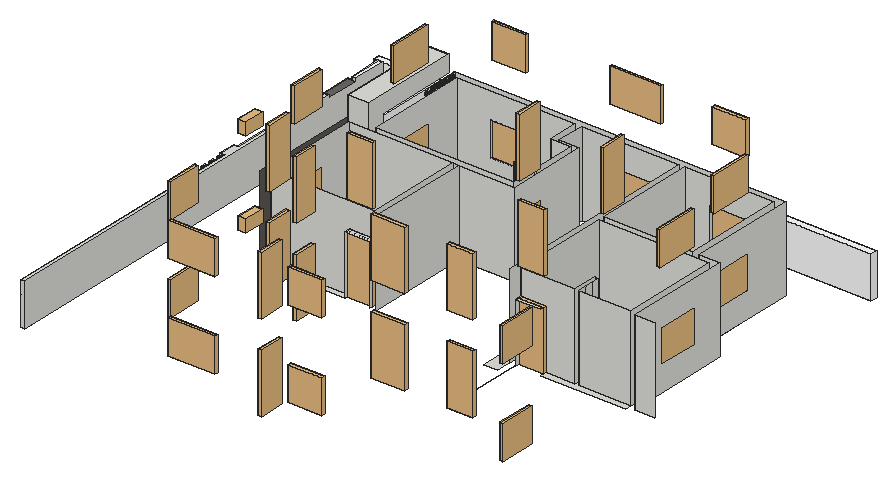
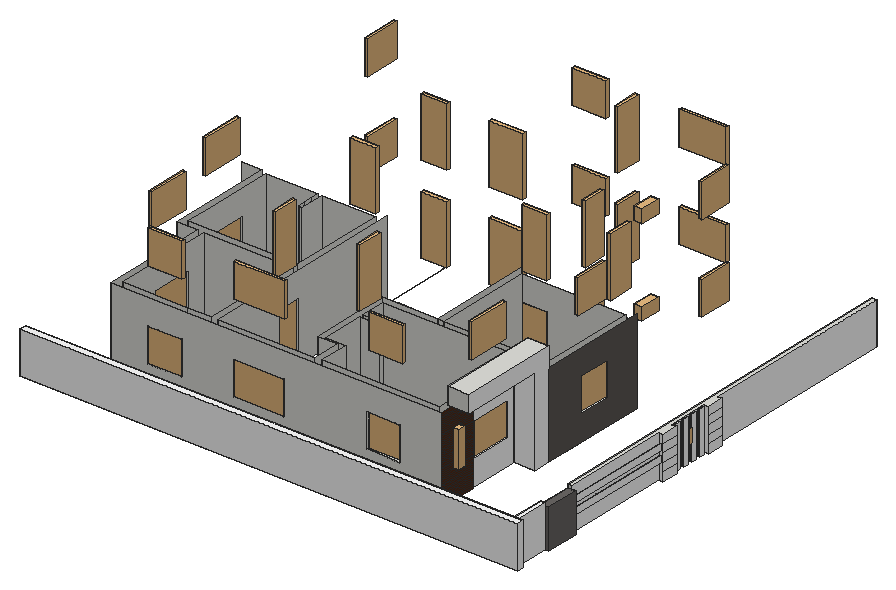
# SketchUp Ruby script. Lengths in inches.
U = 1.inch
M = Sketchup.active_model
def pt(a) = Geom::Point3d.new(a.map { |v| v * U })
def face(e, loops, mat)
  f = e.add_face(loops[0].map { |a| pt(a) })
  loops[1..].each { |l| e.add_face(l.map { |a| pt(a) }).erase! }
  f.material = f.back_material = mat if mat
  f
end
# faces: each face lists its corners as indices into pts; further lists are holes
def faces(e, pts, list, mat = nil) = list.each { |f| face(e, (f[0].is_a?(Array) ? f : [f]).map { |l| l.map { |i| pts[i] } }, mat) }
# xy, xz, yz: faces in a plane at the given z, y or x. An outline is a flat list of corners, or four numbers for a rectangle; further outlines are holes
def ring(l) = l.size == 4 ? [[l[0], l[1]], [l[2], l[1]], [l[2], l[3]], [l[0], l[3]]] : l.each_slice(2).to_a
def flat(e, list, mat, &to3) = list.each { |f| face(e, (f[0].is_a?(Array) ? f : [f]).map { |l| ring(l).map { |u, v| to3.(u, v) } }, mat) }
def xy(e, z, list, mat = nil) = flat(e, list, mat) { |x, y| [x, y, z] }
def xz(e, y, list, mat = nil) = flat(e, list, mat) { |x, z| [x, y, z] }
def yz(e, x, list, mat = nil) = flat(e, list, mat) { |y, z| [x, y, z] }
def lines(e, pts, list) = list.each { |a, b| e.add_line(pt(pts[a]), pt(pts[b])) }
# prism: a flat outline (further loops are holes) pulled along v
def prism(e, loops, v, mat = nil)
  f = face(e, loops, mat); d = Geom::Vector3d.new(v.map { |x| x * U })
  f.pushpull(f.normal.samedirection?(d) ? d.length : -d.length)
end
def box(e, o, s, mat = nil) = prism(e, [[o, [o[0] + s[0], o[1], o[2]], [o[0] + s[0], o[1] + s[1], o[2]], [o[0], o[1] + s[1], o[2]]]], [0, 0, s[2]], mat)
def at(x, y, z, deg = 0) = Geom::Transformation.translation(pt([x, y, z])) * Geom::Transformation.rotation(ORIGIN, Z_AXIS, deg.degrees)
def axes(o, x, y, z) = Geom::Transformation.new([*x, 0, *y, 0, *z, 0, *pt(o).to_a, 1])
def part(name) = M.definitions.add(name)
# library, detail: a bought-in or finely detailed component or shape, given as its bounding box
def library(name, o, s) = part(name).tap { |d| box(d.entities, o, s) }
def detail(e, o, s) = box(e.add_group.entities, o, s)
def put(e, d, t, mat = nil) = e.add_instance(d, t).tap { |i| i.material = mat if mat }
def group(e, t, mat = nil) = e.add_group.tap { |g| g.transformation = t; g.material = mat if mat }.entities
root = M.entities
M.materials.add("Bricks A03 100cm").color = [95, 90, 86]
M.materials.add("Cl-3460 22.24cm").color = [255, 255, 255]
M.materials.add("Manhattan Creative Coating MD 1125B 26.44cm").color = [255, 255, 255]
M.materials.add("Paint White Matte 002 0.02cm").color = [255, 255, 255]
M.materials.add("Pp-1846-msg 17.72cm").color = [255, 255, 255]
M.materials.add("Stone C 250cm").color = [107, 104, 102]
M.materials.add("Wintan - wpa36452 29.79cm").color = [255, 255, 255]
M.materials.add("Wintan - wpa36452 29.79cm\#1").color = [255, 255, 255]
M.materials.add("Wood 011 26.84cm").color = [255, 255, 255]
M.materials.add("Wood Mahogany 33-46 100cm").color = [84, 42, 21]
c1 = library("Window Crafter Sliding 3",[0,-0.55,0],[48,4.49,48])
c2 = library("usa interior dubla",[9.3,83.61,0],[74.77,5.52,82.68])
c3 = library("Window Crafter Awning 2",[0,-9.5,0],[29,11.27,18])
c4 = library("Door 243 065",[-19.36,-2.49,0],[38.72,4.98,81.96])
c5 = library("Door 243 074",[-20.11,-2.41,0],[40.22,4.82,86.63])
c6 = part("*U28\#1")
p = [[0,0,0],[0,36,0],[-1.75,36,0],[-1.75,0,0],[-2.26,35.93,0],[-4.51,35.72,0],
  [-6.75,35.36,0],[-8.95,34.87,0],[-11.125,34.24,0],[-13.25,33.47,0],[-15.33,32.57,0],[-17.34,31.55,0],
  [-19.29,30.4,0],[-21.16,29.125,0],[-22.95,27.74,0],[-24.64,26.24,0],[-26.24,24.64,0],[-27.74,22.95,0],
  [-29.125,21.16,0],[-30.4,19.29,0],[-31.55,17.34,0],[-32.57,15.33,0],[-33.47,13.25,0],[-34.24,11.125,0],
  [-34.87,8.95,0],[-35.36,6.75,0],[-35.72,4.51,0],[-35.93,2.26,0],[-36,0,0],[0,-6,0],
  [-36,-6,0]]
lines(c6.entities,p,[[0,1],[1,2],[2,3],[3,0],[1,4],[4,5],[5,6],[6,7],[7,8],[8,9],[9,10],[10,11],
  [11,12],[12,13],[13,14],[14,15],[15,16],[16,17],[17,18],[18,19],[19,20],[20,21],[21,22],[22,23],
  [23,24],[24,25],[25,26],[26,27],[27,28],[0,29],[28,30]])
c7 = part("Rectangular post")
xy(c7.entities,0,[[0,0,3.4375,7.625]])
xy(c7.entities,60,[[0,0,3.4375,7.625]],"Paint White Matte 002 0.02cm")
xz(c7.entities,0,[[0,0,3.4375,60]],"Paint White Matte 002 0.02cm")
xz(c7.entities,7.625,[[0,0,3.4375,60]],"Paint White Matte 002 0.02cm")
yz(c7.entities,0,[[0,0,7.625,60]],"Paint White Matte 002 0.02cm")
yz(c7.entities,3.4375,[[0,0,7.625,60]])
c8 = library("Group\#37",[0,0,0],[10.9375,10.44,50.62])
c9 = part("*U29\#1")
p = [[0,0,0],[0,-36,0],[-1.75,-36,0],[-1.75,0,0],[-36,0,0],[-35.93,-2.26,0],
  [-35.72,-4.51,0],[-35.36,-6.75,0],[-34.87,-8.95,0],[-34.24,-11.125,0],[-33.47,-13.25,0],[-32.57,-15.33,0],
  [-31.55,-17.34,0],[-30.4,-19.29,0],[-29.125,-21.16,0],[-27.74,-22.95,0],[-26.24,-24.64,0],[-24.64,-26.24,0],
  [-22.95,-27.74,0],[-21.16,-29.125,0],[-19.29,-30.4,0],[-17.34,-31.55,0],[-15.33,-32.57,0],[-13.25,-33.47,0],
  [-11.125,-34.24,0],[-8.95,-34.87,0],[-6.75,-35.36,0],[-4.51,-35.72,0],[-2.26,-35.93,0],[0,6,0],
  [-36,6,0]]
lines(c9.entities,p,[[0,1],[1,2],[2,3],[3,0],[4,5],[5,6],[6,7],[7,8],[8,9],[9,10],[10,11],[11,12],
  [12,13],[13,14],[14,15],[15,16],[16,17],[17,18],[18,19],[19,20],[20,21],[21,22],[22,23],[23,24],
  [24,25],[25,26],[26,27],[27,28],[28,1],[0,29],[4,30]])
c10 = part("Group\#34")
box(c10.entities,[0,0,0],[3,153.5625,9])
c11 = library("Dining Set - 36 x 72 in.\#3",[-45.5,-27.5,0],[91,55,0.01])
c12 = library("Range-Oven - 30 in top\#2",[0,-26,0],[30,26,0.01])
xy(root,0,[[511.31,291.22,511.37,550.5],[482.12,382.5,502.31,449.24],[547.31,403.5,547.31,412.5,587.97,412.5,587.97,447.375,592.97,447.375,592.97,412.5,667.31,412.5,667.31,403.5],[148.31,403.63,148.31,454.3,157.31,454.3,157.31,412.5,268.31,412.5,268.31,403.63],[268.31,403.63,268.43,412.5],
  [645.22,465.17,654.6,479.125,654.6,473.03,665.48,473.03,665.48,492.22,655.11,492.22,655.11,496.88,665.48,496.88,665.48,516.07,655.11,516.07,655.11,523.17,667.17,523.17,667.17,465.17],[654.6,479.125,654.6,479.87,655.11,479.87],[640.18,479.87,640.02,480.43,639.96,480.67,640.32,480.3,640.74,479.87],[654.6,479.87,655.11,492.22],[639.96,480.67,639.9,480.74,639.8,480.84,639.73,481,639.51,481.57,639.29,482.13,638.83,483.27,638.6,483.83,638.37,484.4,638.13,484.96,637.89,485.51,637.64,486.07,637.39,486.62,637.14,487.16,636.88,487.7,636.34,488.76,636.0625,489.27,635.78,489.78,635.48,490.29,635.18,490.78,634.875,491.26,634.56,491.73,634.23,492.2,633.89,492.65,633.55,493.08,633.19,493.51,632.83,493.92,632.45,494.32,632.0625,494.7,631.66,495.07,631.25,495.42,630.83,495.75,630.39,496.07,629.9375,496.37,629.47,496.65,628.99,496.92,628.5,497.16,627.99,497.38,627.47,497.59,626.93,497.77,626.38,497.94,625.82,498.09,625.25,498.23,624.68,498.36,623.52,498.6,622.36,498.82,620.65,499.15,619.55,499.41,619.02,499.55,618.51,499.7,618.01,499.87,617.53,500.06,617.07,500.26,616.63,500.49,616.22,500.73,615.83,501.01,615.46,501.3,615.11,501.61,614.79,501.95,614.49,502.31,614.21,502.68,613.94,503.08,613.7,503.49,613.48,503.92,613.27,504.37,613.08,504.84,612.91,505.32,612.76,505.82,612.62,506.33,612.5,506.86,612.39,507.4,612.3,507.95,612.22,508.52,612.15,509.1,612.09,509.7,612.05,510.3,612.02,510.91,611.99,511.54,611.98,512.17,611.98,512.82,611.99,513.47,612,514.13,612.02,514.8,612.05,515.47,612.09,516.15,612.17,517.53,612.23,518.22,612.28,518.92,612.4,520.33,612.47,521.04,612.53,521.75,612.67,523.17,616.25,523.17,616.22,522.54,616.14,521.28,616.1,520.66,616.07,520.03,616.01,518.79,615.99,518.18,615.97,517.5625,615.95,516.95,615.94,516.35,615.94,515.15,615.95,514.5625,615.97,513.98,615.99,513.4,616.03,512.83,616.07,512.27,616.125,511.71,616.1875,511.17,616.26,510.63,616.34,510.1,616.4375,509.58,616.55,509.07,616.67,508.57,616.8,508.08,616.95,507.6,617.11,507.14,617.29,506.68,617.49,506.24,617.69,505.81,617.92,505.4,618.16,505,618.42,504.61,618.7,504.24,619,503.88,619.32,503.54,619.65,503.21,620.01,502.9,620.39,502.61,620.78,502.33,621.2,502.07,621.63,501.82,622.08,501.59,622.55,501.36,623.02,501.14,623.51,500.94,624,500.73,624.5,500.53,625,500.34,625.51,500.14,626.02,499.95,627.04,499.55,627.55,499.34,628.05,499.13,628.54,498.91,629.03,498.6875,629.5,498.45,629.96,498.2,630.41,497.93,630.85,497.65,631.27,497.36,631.67,497.05,632.07,496.73,632.45,496.4,632.8125,496.05,633.17,495.69,633.51,495.32,633.84,494.9375,634.16,494.54,634.47,494.14,634.76,493.72,635.05,493.29,635.33,492.86,635.6,492.41,635.86,491.96,636.11,491.5,636.35,491.02,636.81,490.06,637.03,489.5625,637.24,489.0625,637.45,488.55,637.65,488.04,638.03,487,638.39,485.94,638.57,485.4,638.74,484.86,638.91,484.31,639.07,483.76,639.24,483.21,639.4,482.66,639.56,482.1,639.71,481.55,639.87,480.99],
  [654.6,496.88,655.11,516.07],[148.31,502.3,148.31,559.5,178.31,559.5,178.31,594.58,187.31,594.58,187.31,559.5,392.57,559.5,392.57,550.5,157.31,550.5,157.31,502.3],[392.57,550.5,502.31,559.5],[214.32,559.5,281.06,580.44],[637.31,586.67,646.31,646.67],
  [502.31,595.5,502.31,703.5,473.12,703.5,473.12,712.5,546.3125,712.5,546.3125,703.5,511.31,703.5,511.31,595.5],[355.31,595.72,355.31,600.44,383.57,600.44,383.57,660.44,355.31,660.44,355.31,703.5,284.58,703.5,284.58,712.5,401.12,712.5,401.12,703.5,364.31,703.5,364.31,664.25,392.57,664.25,392.57,595.72],[637.31,646.67,637.31,703.5,594.3125,703.5,594.3125,712.5,646.31,712.5,646.31,646.67],[178.31,654.58,178.31,712.5,236.58,712.5,236.58,703.5,187.31,703.5,187.31,654.58],[401.12,703.5,473.12,712.5],
  [718.31,763.5,727.31,772.5],[373.31,769.5,400.94,772.5],[400.94,769.5,403.94,772.5],[447.58,769.5,450.58,772.5],[450.58,769.5,490.31,772.5]])
xy(root,36,[[667.31,453.9,676.31,513.9],[148.31,454.3,157.31,502.3],[637.31,586.67,646.31,646.67],[178.31,594.58,187.31,654.58],[236.58,703.5,284.58,712.5],
  [401.12,703.5,473.12,712.5],[546.3125,703.5,594.3125,712.5]])
xy(root,84,[[511.31,403.5,547.31,412.5],[268.31,403.63,304.31,412.5],[667.31,453.9,676.31,513.9],[148.31,454.3,157.31,502.3],[383.57,559.5,392.57,595.72],
  [502.31,559.5,511.31,595.5],[637.31,586.67,646.31,646.67],[178.31,594.58,187.31,654.58],[236.58,703.5,284.58,712.5],[401.12,703.5,473.12,712.5],
  [546.3125,703.5,594.3125,712.5]])
xz(root,408.16,[[676.31,0,704.78,120]])
xz(root,412.5,[[157.31,0,157.31,120,304.31,120,304.31,84,268.31,84,268.31,0],[547.31,0,547.31,84,511.31,84,511.31,120,587.97,120,587.97,0],[592.97,0,667.31,120]])
xz(root,447.375,[[587.97,0,592.97,120]])
xz(root,453.9,[[667.31,36,676.31,84]])
xz(root,454.3,[[148.31,36,157.31,84]])
xz(root,502.3,[[148.31,36,157.31,84]])
xz(root,513.9,[[667.31,36,676.31,84]])
xz(root,550.5,[[157.31,0,304.31,120],[304.31,0,313.31,120],[313.31,0,392.57,120],[511.31,0,511.37,120],[511.37,0,667.31,120]])
xz(root,559.5,[[187.31,0,187.31,120,383.57,120,383.57,84,392.57,84,392.57,0],[502.31,0,502.31,84,511.31,84,511.31,120,637.31,120,637.31,0],[646.31,0,676.31,120]])
xz(root,559.5,[[148.31,0,178.31,120]],"Pp-1846-msg 17.72cm")
xz(root,586.67,[[637.31,36,646.31,84]])
xz(root,594.58,[[178.31,36,187.31,84]])
xz(root,595.5,[[502.31,0,511.31,84]])
xz(root,595.72,[[355.31,0,392.57,0,392.57,84,383.57,84,383.57,120,355.31,120]])
xz(root,600.44,[[355.31,0,383.57,120]])
xz(root,646.67,[[637.31,36,646.31,84]])
xz(root,654.58,[[178.31,36,187.31,84]])
xz(root,660.44,[[355.31,0,383.57,120]])
xz(root,664.25,[[364.31,0,392.57,120]])
xz(root,703.5,[[[187.31,0,355.31,120],[236.58,36,284.58,84]],[[364.31,0,502.31,120],[401.12,36,473.12,84]],[511.31,0,546.3125,120],[546.3125,0,594.3125,36],[594.3125,0,637.31,0,637.31,120,546.3125,120,546.3125,84,594.3125,84]])
xz(root,712.5,[[[178.31,0,646.31,120],[401.12,36,473.12,84],[236.58,36,284.58,84],[546.3125,36,594.3125,84]]])
yz(root,148.31,[[[403.63,0,559.5,120],[454.3,36,502.3,84]]],"Bricks A03 100cm")
yz(root,157.31,[[412.5,0,454.3,0,454.3,84,502.3,84,502.3,36,454.3,36,454.3,0,550.5,0,550.5,120,412.5,120]])
yz(root,178.31,[[[559.5,0,712.5,120],[594.58,36,654.58,84]]],"Pp-1846-msg 17.72cm")
yz(root,187.31,[[[559.5,0,703.5,120],[594.58,36,654.58,84]]])
yz(root,236.58,[[703.5,36,712.5,84]])
yz(root,268.31,[[403.63,0,412.5,84]])
yz(root,284.58,[[703.5,36,712.5,84]])
yz(root,304.31,[[403.63,0,403.63,84,412.5,84,412.5,120,550.5,120,550.5,0]])
yz(root,313.31,[[403.63,0,550.5,120]])
yz(root,355.31,[[595.72,0,600.44,120],[660.44,0,703.5,120]])
yz(root,364.31,[[664.25,0,703.5,120]])
yz(root,383.57,[[600.44,0,660.44,120],[559.5,84,595.72,120]])
yz(root,392.57,[[550.5,0,559.5,0,559.5,84,595.72,84,595.72,0,664.25,0,664.25,120,550.5,120]])
yz(root,401.12,[[703.5,36,712.5,84]])
yz(root,473.12,[[703.5,36,712.5,84]])
yz(root,502.31,[[403.5,0,403.5,120,703.5,120,703.5,0,595.5,0,595.5,84,559.5,84,559.5,0]])
yz(root,511.31,[[403.5,0,550.5,0,550.5,120,412.5,120,412.5,84,403.5,84],[595.5,0,703.5,0,703.5,120,559.5,120,559.5,84,595.5,84]])
yz(root,546.3125,[[703.5,36,712.5,84]])
yz(root,587.97,[[412.5,0,447.375,120]])
yz(root,592.97,[[412.5,0,424.8,120],[424.8,0,437.1,120],[437.1,0,447.375,120]])
yz(root,594.3125,[[703.5,36,712.5,84]])
yz(root,637.31,[[[559.5,0,703.5,120],[586.67,36,646.67,84]]])
yz(root,646.31,[[[559.5,0,712.5,120],[586.67,36,646.67,84]]])
yz(root,667.31,[[412.5,0,412.5,120,513.9,120,513.9,84,453.9,84,453.9,36,513.9,36,513.9,120,550.5,120,550.5,0]])
yz(root,676.31,[[[408.16,0,559.5,120],[453.9,36,513.9,84]]])
g1 = group(root,at(152.26,130.41,-0.07))
put(g1,c1,at(394.05,577.59,36.07))
put(g1,c1,at(84.32,574.2,36.07))
put(g1,c1,at(32.24,69.17,36.07,90))
put(g1,c1,at(3.9375,323.89,36.07,90))
put(g1,c1,axes([248.86,577.59,36.07],[1.5,0,0],[0,1,0],[0,0,1]))
put(g1,c1,axes([33.3125,464.17,36.07],[0,1.25,0],[-1,0,0],[0,0,1]))
put(g1,c1,axes([84.3,0.55,36.07],[1.3875,0,0],[0,1,0],[0,0,1]))
put(g1,c1,axes([492.9375,456.26,36.07],[0,1.25,0],[-1,0,0],[0,0,1]))
put(g1,c1,axes([522.9375,323.5,36.07],[0,1.25,0],[-1,0,0],[0,0,1]))
put(g1,c1,axes([522.9375,45.26,36.07],[0,1.0625,0],[-1,0,0],[0,0,1]))
put(g1,c2,axes([245.08,62.12,0.07],[0.64285,0,0],[0,1.06,0],[0,0,1.016]))
put(g1,c3,at(30.9,232.09,84.07,-90))
put(g1,c4,axes([376.95,280.08,0.07],[0.93479,0,0],[0,1,0],[0,0,1.02567]))
put(g1,c4,axes([376.95,154.08,0.07],[0.93479,0,0],[0,1,0],[0,0,1.02567]))
put(g1,c4,axes([208.75,25.49,0.07],[0,-0.93479,0],[1,0,0],[0,0,1.02567]))
put(g1,c4,axes([134.02,280.14,0],[0.93134,0,0],[0,1,0],[0,0,1.02567]))
put(g1,c5,axes([104.21,216.125,0],[0,0.7938,0],[-1,0,0],[0,0,0.97036]))
put(g1,c4,axes([237.01,447.21,0.07],[0,-0.93479,0],[1,0,0],[0,0,1.02567]))
put(g1,c4,axes([35.97,255.12,0],[0,-0.93479,0],[1,0,0],[0,0,1.02567]))
put(g1,c4,axes([356.57,447.21,0.07],[0,-0.93479,0],[1,0,0],[0,0,1.02567]))
g2 = group(root,at(152.26,130.41,123.93))
put(g2,c1,at(394.05,577.59,36.07))
put(g2,c1,at(84.32,574.2,36.07))
put(g2,c1,at(32.24,69.17,36.07,90))
put(g2,c1,at(3.9375,323.89,36.07,90))
put(g2,c1,axes([248.86,577.59,36.07],[1.5,0,0],[0,1,0],[0,0,1]))
put(g2,c1,axes([33.3125,464.17,36.07],[0,1.25,0],[-1,0,0],[0,0,1]))
put(g2,c1,axes([84.3,0.55,36.07],[1.3875,0,0],[0,1,0],[0,0,1]))
put(g2,c1,axes([492.9375,456.26,36.07],[0,1.25,0],[-1,0,0],[0,0,1]))
put(g2,c1,axes([522.9375,323.5,36.07],[0,1.25,0],[-1,0,0],[0,0,1]))
put(g2,c1,axes([522.9375,45.26,36.07],[0,1.0625,0],[-1,0,0],[0,0,1]))
put(g2,c2,axes([245.08,62.12,0.07],[0.64285,0,0],[0,1.06,0],[0,0,1.016]))
put(g2,c3,at(30.9,232.09,84.07,-90))
put(g2,c4,axes([376.95,280.08,0.07],[0.93479,0,0],[0,1,0],[0,0,1.02567]))
put(g2,c4,axes([376.95,154.08,0.07],[0.93479,0,0],[0,1,0],[0,0,1.02567]))
put(g2,c4,axes([208.75,25.49,0.07],[0,-0.93479,0],[1,0,0],[0,0,1.02567]))
put(g2,c4,axes([134.02,280.14,0],[0.93134,0,0],[0,1,0],[0,0,1.02567]))
put(g2,c5,axes([104.21,216.125,0],[0,0.7938,0],[-1,0,0],[0,0,0.97036]))
put(g2,c4,axes([237.01,447.21,0.07],[0,-0.93479,0],[1,0,0],[0,0,1.02567]))
put(g2,c4,axes([35.97,255.12,0],[0,-0.93479,0],[1,0,0],[0,0,1.02567]))
put(g2,c4,axes([356.57,447.21,0.07],[0,-0.93479,0],[1,0,0],[0,0,1.02567]))
put(g2,c1,at(302.05,4.78,36.07,-180))
put(g2,c1,at(302.05,4.9,-87.93,-180))
put(root,c6,at(304.43,409.63,0))
put(root,c6,axes([511.37,411.39,0],[-1,0,0],[0,1,0],[0,0,1]))
put(root,c7,at(24.87,438.5,0))
g3 = group(root,at(28.31,129,0))
xy(g3,0,[[0,0,0,280.875,-6,280.875,-6,304.875,0,304.875,0,539.4375,-6,539.4375,-6,587.4375,0,587.4375,0,634.5,6,634.5,6,0],[-6,361.875,0,385.875]])
xy(g3,55.875,[[-6,539.4375,6,587.4375]],"Stone C 250cm")
xy(g3,60,[[0,0,6,0,6,539.4375,0,539.4375,0,385.875,-6,385.875,-6,361.875,0,361.875,0,304.875,-6,304.875,-6,280.875,0,280.875]])
xy(g3,60,[[0,587.4375,6,634.5]],"Cl-3460 22.24cm")
xz(g3,0,[[0,0,6,60]])
xz(g3,280.875,[[-6,0,0,60]],"Wintan - wpa36452 29.79cm\#1")
xz(g3,304.875,[[-6,0,0,60]],"Wintan - wpa36452 29.79cm\#1")
xz(g3,361.875,[[-6,0,0,60]],"Wintan - wpa36452 29.79cm\#1")
xz(g3,385.875,[[-6,0,0,60]],"Wintan - wpa36452 29.79cm\#1")
xz(g3,539.4375,[[0,55.875,6,60]])
xz(g3,539.4375,[[-6,0,0,55.875]],"Stone C 250cm")
xz(g3,587.4375,[[0,55.875,6,60]])
xz(g3,587.4375,[[-6,0,0,55.875]],"Stone C 250cm")
xz(g3,634.5,[[0,0,6,60]])
yz(g3,-6,[[539.4375,0,587.4375,55.875]],"Stone C 250cm")
yz(g3,-6,[[280.875,0,304.875,12],[361.875,0,385.875,12],[280.875,12,304.875,24],[361.875,12,385.875,24],[280.875,24,304.875,36],
  [361.875,24,385.875,36],[280.875,36,304.875,48],[361.875,36,385.875,48],[280.875,48,304.875,60],[361.875,48,385.875,60]],"Wintan - wpa36452 29.79cm\#1")
yz(g3,0,[[0,0,280.875,60],[385.875,0,539.4375,60],[587.4375,0,634.5,60]],"Cl-3460 22.24cm")
yz(g3,0,[[304.875,0,361.875,60]],"Wood 011 26.84cm")
yz(g3,6,[[0,0,634.5,0,634.5,60,587.4375,60,587.4375,55.875,539.4375,55.875,539.4375,60,0,60]])
put(root,c7,at(24.87,452.6875,0))
put(root,c8,axes([24.43,461.26,24.77],[0.38,0,0],[0,0.38,0],[0,0,0.38]))
put(root,c7,at(24.87,466.875,0))
put(root,c7,at(24.87,481.0625,0))
put(root,c9,axes([508.37,559.5,0],[0,-1,0],[-1,0,0],[0,0,1]))
put(root,c10,at(25.31,514.875,22.59),"Manhattan Creative Coating MD 1125B 26.44cm")
put(root,c10,at(25.31,514.875,37.59),"Manhattan Creative Coating MD 1125B 26.44cm")
put(root,c11,axes([444.8,625.02,0],[0.79513,0,0],[0,0.79513,0],[0,0,0.79513]))
g4 = group(root,at(148.31,559.5,0))
xy(g4,0,[[0,0,30,24]])
xy(g4,124,[[0,24,30,141]])
xy(g4,148,[[0,0,30,141]])
xz(g4,0,[[0,0,30,148]])
xz(g4,24,[[0,0,30,124]],"Pp-1846-msg 17.72cm")
xz(g4,141,[[0,124,30,148]])
yz(g4,0,[[0,0,0,148,141,148,141,124,24,124,24,0]],"Wintan - wpa36452 29.79cm")
yz(g4,30,[[0,0,24,0,24,124,141,124,141,148,0,148]])
g5 = group(root,at(177.31,658.33,0),"Wood Mahogany 33-46 100cm")
prism(g5,[[[1,0,0],[1,0,120],[0,0,120],[0,0,117.6],[0,0,115.2],[0,0,112.8],[0,0,110.4],[0,0,108],[0,0,105.6],[0,0,103.2],[0,0,100.8],[0,0,98.4],[0,0,96],[0,0,93.6],[0,0,91.2],[0,0,88.8],[0,0,86.4],[0,0,84],[0,0,81.6],[0,0,79.2],[0,0,76.8],[0,0,74.4],[0,0,72],[0,0,69.6],[0,0,67.2],[0,0,64.8],[0,0,62.4],[0,0,60],[0,0,57.6],[0,0,55.2],[0,0,52.8],[0,0,50.4],[0,0,48],[0,0,45.6],[0,0,43.2],[0,0,40.8],[0,0,38.4],[0,0,36],[0,0,33.6],[0,0,31.2],[0,0,28.8],[0,0,26.4],[0,0,24],[0,0,21.6],[0,0,19.2],[0,0,16.8],[0,0,14.4],[0,0,12],[0,0,9.6],[0,0,7.2],[0,0,4.8],[0,0,2.4],[0,0,0]]],[0,54.17,0],"Wood Mahogany 33-46 100cm")
put(root,c8,at(168.06,683.21,42.42))
put(root,c12,at(555.92,703.83,0))
g6 = group(root,at(22.31,763.5,0),"Pp-1846-msg 17.72cm")
box(g6,[0,0,0],[705,9,60])
